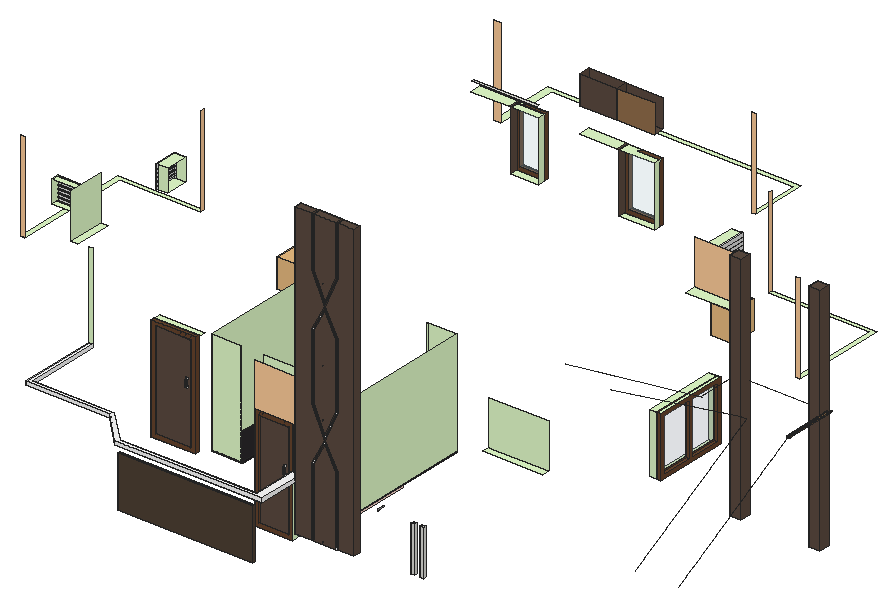
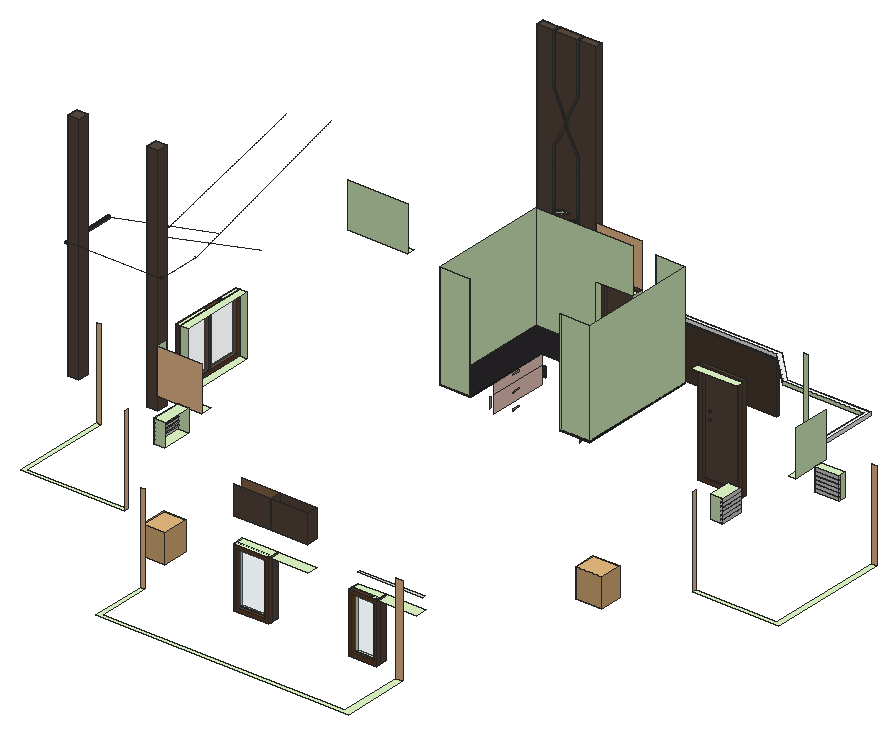
# SketchUp Ruby script. Lengths in inches.
U = 1.inch
M = Sketchup.active_model
def pt(a) = Geom::Point3d.new(a.map { |v| v * U })
def face(e, loops, mat)
  f = e.add_face(loops[0].map { |a| pt(a) })
  loops[1..].each { |l| e.add_face(l.map { |a| pt(a) }).erase! }
  f.material = f.back_material = mat if mat
  f
end
# faces: each face lists its corners as indices into pts; further lists are holes
def faces(e, pts, list, mat = nil) = list.each { |f| face(e, (f[0].is_a?(Array) ? f : [f]).map { |l| l.map { |i| pts[i] } }, mat) }
# xy, xz, yz: faces in a plane at the given z, y or x. An outline is a flat list of corners, or four numbers for a rectangle; further outlines are holes
def ring(l) = l.size == 4 ? [[l[0], l[1]], [l[2], l[1]], [l[2], l[3]], [l[0], l[3]]] : l.each_slice(2).to_a
def flat(e, list, mat, &to3) = list.each { |f| face(e, (f[0].is_a?(Array) ? f : [f]).map { |l| ring(l).map { |u, v| to3.(u, v) } }, mat) }
def xy(e, z, list, mat = nil) = flat(e, list, mat) { |x, y| [x, y, z] }
def xz(e, y, list, mat = nil) = flat(e, list, mat) { |x, z| [x, y, z] }
def yz(e, x, list, mat = nil) = flat(e, list, mat) { |y, z| [x, y, z] }
def lines(e, pts, list) = list.each { |a, b| e.add_line(pt(pts[a]), pt(pts[b])) }
# prism: a flat outline (further loops are holes) pulled along v
def prism(e, loops, v, mat = nil)
  f = face(e, loops, mat); d = Geom::Vector3d.new(v.map { |x| x * U })
  f.pushpull(f.normal.samedirection?(d) ? d.length : -d.length)
end
def box(e, o, s, mat = nil) = prism(e, [[o, [o[0] + s[0], o[1], o[2]], [o[0] + s[0], o[1] + s[1], o[2]], [o[0], o[1] + s[1], o[2]]]], [0, 0, s[2]], mat)
def at(x, y, z, deg = 0) = Geom::Transformation.translation(pt([x, y, z])) * Geom::Transformation.rotation(ORIGIN, Z_AXIS, deg.degrees)
def axes(o, x, y, z) = Geom::Transformation.new([*x, 0, *y, 0, *z, 0, *pt(o).to_a, 1])
def part(name) = M.definitions.add(name)
# library, detail: a bought-in or finely detailed component or shape, given as its bounding box
def library(name, o, s) = part(name).tap { |d| box(d.entities, o, s) }
def detail(e, o, s) = box(e.add_group.entities, o, s)
def put(e, d, t, mat = nil) = e.add_instance(d, t).tap { |i| i.material = mat if mat }
def group(e, t, mat = nil) = e.add_group.tap { |g| g.transformation = t; g.material = mat if mat }.entities
root = M.entities
M.materials.add("Asphalt_01_1K").color = [79, 65, 53]
M.materials.add("B01_Ivory_Dust").color = [255, 217, 206]
M.materials.add("C02_Golden_Beige").color = [255, 205, 155]
M.materials.add("F01_Seafoam_Drift").color = [229, 255, 204]
M.materials.add("Glass_Basic_01").color = [161, 173, 186]
M.materials["Glass_Basic_01"].alpha = 0.25
M.materials.add("Glass_Safety_01").color = [204, 235, 244]
M.materials["Glass_Safety_01"].alpha = 0.25
M.materials.add("M00_Soft_Cloud").color = [255, 255, 255]
M.materials.add("M01_Silver_Fog").color = [224, 224, 224]
M.materials.add("M03_Pewter_Shine").color = [168, 168, 168]
M.materials.add("M06_Steel_Smoke").color = [86, 86, 86]
M.materials.add("M08_Obsidian_Black").color = [30, 30, 30]
M.materials.add("M09_Shadow_Night").color = [0, 0, 0]
M.materials.add("Marble_07_1K").color = [36, 34, 36]
M.materials.add("Metal_06_1K").color = [238, 236, 231]
M.materials.add("Plywood_01_1K").color = [125, 96, 64]
M.materials.add("Wood_Floor_01_1K").color = [146, 111, 76]
M.materials.add("Wood_Floor_12_1K").color = [92, 75, 65]
M.materials.add("Wood_Veneer_15_1K").color = [103, 69, 45]
c1 = part("Group\#25")
xy(c1.entities,0,[[0,-3,30,0]],"Wood_Veneer_15_1K")
xy(c1.entities,3,[[3,-2.25,27,0]],"Wood_Floor_12_1K")
xy(c1.entities,3,[[3,-3,27,-2.25]],"Wood_Veneer_15_1K")
xy(c1.entities,81,[[3,-2.25,27,0]],"Wood_Floor_12_1K")
xy(c1.entities,81,[[3,-3,27,-2.25]],"Wood_Veneer_15_1K")
xy(c1.entities,84,[[0,-3,30,0]],"Wood_Veneer_15_1K")
xz(c1.entities,-3,[[[0,0,30,84],[3,3,27,81]]],"Wood_Veneer_15_1K")
xz(c1.entities,-2.25,[[3,3,27,81]],"Wood_Floor_12_1K")
xz(c1.entities,0,[[[0,0,30,84],[3,3,27,81]]],"Wood_Veneer_15_1K")
yz(c1.entities,0,[[-3,0,0,84]],"Wood_Veneer_15_1K")
yz(c1.entities,3,[[-2.25,3,0,81]],"Wood_Floor_12_1K")
yz(c1.entities,3,[[-3,3,-2.25,81]],"Wood_Veneer_15_1K")
yz(c1.entities,27,[[-2.25,3,0,81]],"Wood_Floor_12_1K")
yz(c1.entities,27,[[-3,3,-2.25,81]],"Wood_Veneer_15_1K")
yz(c1.entities,30,[[-3,0,0,84]],"Wood_Veneer_15_1K")
g1 = group(c1.entities,at(22.875,-2.25,50.47),"Metal_06_1K")
xy(g1,-5.5625,[[0,-0.48,1.25,0]],"Metal_06_1K")
xy(g1,-4.9375,[[0,-1.375,1.25,-0.48]],"Metal_06_1K")
xy(g1,-4.6875,[[0,-1.125,1.25,0]],"Metal_06_1K")
xy(g1,-4.6875,[[0,-1.375,1.25,-1.125]],"Wood_Veneer_15_1K")
xy(g1,0,[[0,-1.125,1.25,-0.5],[0,-0.5,1.25,0]],"Metal_06_1K")
xy(g1,0.25,[[0,-1.375,1.25,-1.125],[0,-1.125,1.25,-0.5]],"Metal_06_1K")
xy(g1,0.25,[[0,-0.5,1.25,0]],"Wood_Veneer_15_1K")
xy(g1,1.25,[[0,-0.5,1.25,0]],"Metal_06_1K")
xz(g1,-1.375,[[0,-4.9375,1.25,-4.6875],[0,-4.6875,1.25,0.25]],"Metal_06_1K")
xz(g1,-1.125,[[0,-4.6875,1.25,0],[0,0,1.25,0.25]],"Metal_06_1K")
xz(g1,-0.5,[[0,0.25,1.25,1.25]],"Metal_06_1K")
xz(g1,-0.5,[[0,0,1.25,0.25]],"Wood_Veneer_15_1K")
xz(g1,-0.48,[[0,-5.5625,1.25,-4.9375]],"Metal_06_1K")
xz(g1,0,[[0,0.25,1.25,1.25]],"Metal_06_1K")
xz(g1,0,[[0,-5.5625,1.25,-4.6875],[0,0,1.25,0.25]],"Wood_Veneer_15_1K")
yz(g1,0,[[-0.48,-5.5625,-0.48,-4.9375,-1.375,-4.9375,-1.375,-4.6875,0,-4.6875,0,-5.5625],[-1.375,-4.6875,-1.125,0.25],[-1.125,0,-0.5,0.25],[-0.5,0,0,0.25],[-0.5,0.25,0,1.25]],"Metal_06_1K")
yz(g1,1.25,[[-0.48,-5.5625,0,-5.5625,0,-4.6875,-1.375,-4.6875,-1.375,-4.9375,-0.48,-4.9375],[-1.375,-4.6875,-1.125,0.25],[-1.125,0,-0.5,0.25],[-0.5,0,0,0.25],[-0.5,0.25,0,1.25]],"Metal_06_1K")
c2 = part("Group\#51")
box(c2.entities,[0,0,-60],[9,9,187])
c3 = part("Group\#15")
box(c3.entities,[0,0,0],[5.9375,1,0.1875],"M03_Pewter_Shine")
c4 = part("Group\#49")
box(c4.entities,[2.9375,2.5,0],[1.8125,1.9375,1.6875],"M09_Shadow_Night")
c5 = part("Group\#58")
xy(c5.entities,0,[[-0.5,0,1.125,43.8125]],"M00_Soft_Cloud")
c6 = part("Group\#67")
box(c6.entities,[0,-2.3125,0],[2.875,2.3125,36.5625])
c7 = library("Hospital Sink 001",[-10.61,-17.4375,27.15],[21.22,17.43,22.96])
c8 = part("Group\#13")
box(c8.entities,[0,0,0],[1.125,8.25,0.1875],"M03_Pewter_Shine")
c9 = part("Group\#17")
xy(c9.entities,0,[[0,0,1.3125,6.9375]],"M06_Steel_Smoke")
c10 = part("Group\#16")
box(c10.entities,[0,0,0],[1.1875,8,0.25],"M03_Pewter_Shine")
c11 = part("Group\#14")
box(c11.entities,[0,0,0],[5.9375,1,0.1875],"M03_Pewter_Shine")
c12 = part("Group\#12")
box(c12.entities,[0,0,0],[5.9375,1,0.1875],"M03_Pewter_Shine")
c13 = part("Group\#28")
xy(c13.entities,0,[[0,0,28.0625,3]],"Wood_Veneer_15_1K")
xy(c13.entities,3,[[3,0,25.0625,3]],"Wood_Veneer_15_1K")
xy(c13.entities,45,[[3,0,25.0625,3]],"Wood_Veneer_15_1K")
xy(c13.entities,48,[[0,0,28.0625,3]],"Wood_Veneer_15_1K")
xz(c13.entities,0,[[3,3,25.0625,45]],"Glass_Safety_01")
xz(c13.entities,0,[[[0,0,28.0625,48],[3,3,25.0625,45]]],"Wood_Veneer_15_1K")
xz(c13.entities,3,[[[0,0,28.0625,48],[3,3,25.0625,45]]],"Wood_Veneer_15_1K")
yz(c13.entities,0,[[0,0,3,48]],"Wood_Veneer_15_1K")
yz(c13.entities,3,[[0,3,3,45]],"Wood_Veneer_15_1K")
yz(c13.entities,25.0625,[[0,3,3,45]],"Wood_Veneer_15_1K")
yz(c13.entities,28.0625,[[0,0,3,48]],"Wood_Veneer_15_1K")
c14 = part("Group\#27")
xy(c14.entities,0,[[0,0,3,60]],"Wood_Veneer_15_1K")
xy(c14.entities,3,[[0,3,3,29],[0,29,3,31],[0,31,3,57]],"Wood_Veneer_15_1K")
xy(c14.entities,45,[[0,3,3,29],[0,31,3,57]],"Wood_Veneer_15_1K")
xy(c14.entities,48,[[0,0,3,60]],"Wood_Veneer_15_1K")
xz(c14.entities,0,[[0,0,3,48]],"Wood_Veneer_15_1K")
xz(c14.entities,3,[[0,3,3,45]],"Wood_Veneer_15_1K")
xz(c14.entities,29,[[0,3,3,45]],"Wood_Veneer_15_1K")
xz(c14.entities,31,[[0,3,3,45]],"Wood_Veneer_15_1K")
xz(c14.entities,57,[[0,3,3,45]],"Wood_Veneer_15_1K")
xz(c14.entities,60,[[0,0,3,48]],"Wood_Veneer_15_1K")
yz(c14.entities,0,[[3,3,29,45],[31,3,57,45]],"Glass_Basic_01")
yz(c14.entities,0,[[[0,0,60,48],[3,3,57,3,57,45,31,45,31,3,29,3,29,45,3,45]]],"Wood_Veneer_15_1K")
yz(c14.entities,3,[[[0,0,60,48],[3,3,3,45,29,45,29,3,31,3,31,45,57,45,57,3]]],"Wood_Veneer_15_1K")
c15 = part("Group\#29")
xy(c15.entities,0,[[0,0,1,24]])
xy(c15.entities,2.6,[[0,0,1,24]])
xy(c15.entities,3,[[0,0,1,24]])
xy(c15.entities,5.6,[[0,0,1,24]])
xy(c15.entities,6,[[0,0,1,24]])
xy(c15.entities,8.6,[[0,0,1,24]])
xy(c15.entities,9,[[0,0,1,24]])
xy(c15.entities,11.6,[[0,0,1,24]])
xy(c15.entities,12,[[0,0,1,24]])
xy(c15.entities,14.6,[[0,0,1,24]])
xy(c15.entities,15,[[0,0,1,24]])
xy(c15.entities,18,[[0,0,1,24]])
xz(c15.entities,0,[[0,0,1,2.6],[0,3,1,5.6],[0,6,1,8.6],[0,9,1,11.6],[0,12,1,14.6],
  [0,15,1,18]])
xz(c15.entities,24,[[0,0,1,2.6],[0,3,1,5.6],[0,6,1,8.6],[0,9,1,11.6],[0,12,1,14.6],
  [0,15,1,18]])
yz(c15.entities,0,[[0,2.6,24,3],[0,5.6,24,6],[0,8.6,24,9],[0,11.6,24,12],[0,14.6,24,15]])
yz(c15.entities,1,[[0,0,24,2.6],[0,3,24,5.6],[0,6,24,8.6],[0,9,24,11.6],[0,12,24,14.6],
  [0,15,24,18]])
xy(root,23,[[1767.92,714.6875,1797.92,723.6875]],"Wood_Floor_12_1K")
xy(root,33.35,[[1804.92,714.6875,1851.8125,715.3125]],"F01_Seafoam_Drift")
xy(root,57,[[1797.92,723.6875,1797.92,747.03,1797.9375,747.22,1797.97,747.41,1798.04,747.59,1798.08,747.6875,1821.8125,747.6875,1821.8125,819.65,1821.81,819.65,1821.96,819.68,1822.1,819.6875,1845.8125,819.6875,1845.8125,723.6875],[1797.92,747.03,1797.9375,747.22,1797.97,747.41,1798.04,747.59,1798.08,747.6875,1797.92,747.6875]],"B01_Ivory_Dust")
xy(root,57,[[1798.08,747.6875,1798.12,747.76,1798.23,747.92,1798.36,748.07,1798.5,748.2,1798.66,748.3,1798.83,748.39,1799.02,748.45,1799.2,748.49,1799.4,748.5,1821,748.5,1821,747.6875],[1821,747.6875,1821.8125,795.6875],[1821,795.6875,1821,818.59,1821.01,818.73,1821.04,818.87,1821.08,819.01,1821.15,819.14,1821.23,819.26,1821.32,819.37,1821.43,819.46,1821.55,819.54,1821.68,819.6,1821.8125,819.65,1821.8125,795.6875],[1821.81,819.65,1821.96,819.68,1822.1,819.6875,1821.8125,819.6875,1821.8125,819.65]],"Marble_07_1K")
xy(root,58,[[1725.8125,723.6875,1725.8125,819.6875,1748.87,819.6875,1749.1,819.67,1749.32,819.63,1749.54,819.55,1749.75,819.45,1749.8125,819.41,1749.8125,723.73,1749.79,723.73,1749.64,723.7,1749.5,723.6875],[1749.5,723.6875,1749.8125,723.6875,1749.8125,723.73,1749.79,723.73,1749.64,723.7]],"B01_Ivory_Dust")
xy(root,58,[[1959.8125,869.89,1968.8125,929.89],[1651.0625,1117.375,1673.1875,1126.375],[1737.77,1117.375,1765.83,1126.375]],"F01_Seafoam_Drift")
xy(root,58,[[1797.92,723.6875,1845.8125,723.6875,1845.8125,819.6875,1822.1,819.6875,1821.96,819.68,1821.81,819.65,1821.68,819.6,1821.55,819.54,1821.43,819.46,1821.32,819.37,1821.23,819.26,1821.15,819.14,1821.08,819.01,1821.04,818.87,1821.01,818.73,1821,818.59,1821,748.5,1799.4,748.5,1799.2,748.49,1799.02,748.45,1798.83,748.39,1798.66,748.3,1798.5,748.2,1798.36,748.07,1798.23,747.92,1798.12,747.76,1798.04,747.59,1797.97,747.41,1797.9375,747.22,1797.92,747.03],[1749.8125,723.73,1749.8125,747.6875,1750.625,747.6875,1750.625,724.82,1750.62,724.67,1750.59,724.52,1750.54,724.38,1750.47,724.25,1750.39,724.13,1750.29,724.02,1750.18,723.92,1750.06,723.84,1749.93,723.77],[1749.8125,747.6875,1750.625,771.6875],[1749.8125,771.6875,1750.625,795.6875],[1749.8125,795.6875,1749.8125,819.41,1749.9375,819.32,1750.11,819.17,1750.26,819,1750.39,818.81,1750.49,818.6,1750.57,818.38,1750.61,818.16,1750.625,817.93,1750.625,795.6875],
  [1749.8125,819.41,1749.8125,819.6875,1748.87,819.6875,1749.1,819.67,1749.32,819.63,1749.54,819.55,1749.75,819.45]],"Marble_07_1K")
xy(root,59,[[1725.8125,723.6875,1749.5,723.6875,1749.64,723.7,1749.79,723.73,1749.93,723.77,1750.06,723.84,1750.18,723.92,1750.29,724.02,1750.39,724.13,1750.47,724.25,1750.54,724.38,1750.59,724.52,1750.62,724.67,1750.625,724.82,1750.625,817.93,1750.61,818.16,1750.57,818.38,1750.49,818.6,1750.39,818.81,1750.26,819,1750.11,819.17,1749.9375,819.32,1749.75,819.45,1749.54,819.55,1749.32,819.63,1749.1,819.67,1748.87,819.6875,1725.8125,819.6875]],"Marble_07_1K")
xy(root,70,[[1687.27,675.6875,1662.78,700.375,1596.1,700.375,1596.1,763.375,1599.1,763.375,1599.1,703.375,1664.03,703.375,1688.52,678.6875,1797.92,678.6875,1797.92,714.6875,1804.92,714.6875,1804.92,675.6875],[1473.8125,847.375,1477.8125,847.375,1477.8125,941.875,1542.8125,941.875,1542.8125,944.875,1473.8125,944.875],[1965.8125,1009.375,1968.8125,1009.375,1968.8125,1086,1884.8125,1086,1884.8125,1083,1965.8125,1083],[1613.1875,1147.375,1619.1875,1147.375,1619.1875,1198.375,1812.8125,1198.375,1812.8125,1156.375,1815.8125,1156.375,1815.8125,1201.375,1613.1875,1201.375]],"F01_Seafoam_Drift")
xy(root,73,[[1687.27,675.6875,1804.92,675.6875,1804.92,714.6875,1797.92,714.6875,1797.92,678.6875,1688.52,678.6875,1664.03,703.375,1599.1,703.375,1599.1,763.375,1596.1,763.375,1596.1,700.375,1662.78,700.375]],"M00_Soft_Cloud")
xy(root,106,[[1767.92,714.6875,1797.92,723.6875],[1911.8125,763,1959.8125,769],[1645.59,763.375,1681.59,772.375],[1542.8125,811.375,1548.8125,841.375],[1504.12,841.375,1523.47,847.375],
  [1959.8125,869.89,1968.8125,929.89],[1542.8125,897.17,1551.8125,915.375],[1875.8125,1033.59,1884.8125,1057.59],[1619.1875,1117.375,1649.1875,1126.375],[1651.0625,1117.375,1673.1875,1126.375],
  [1705.83,1117.375,1735.83,1126.375],[1737.77,1117.375,1765.83,1126.375]],"F01_Seafoam_Drift")
xy(root,106,[[1649.1875,1117.375,1651.0625,1126.375],[1735.83,1117.375,1737.77,1126.375]],"Wood_Floor_12_1K")
xy(root,106.25,[[1884.8125,1000.375,1920.8125,1009.375]],"F01_Seafoam_Drift")
xy(root,123,[[1993.5,912.38,1994.68,912.38,1994.68,912.82,1994.875,912.82,1994.875,914,1993.5,914],[1994.68,912.38,1994.875,912.82],[2066.875,912.38,2067.19,912.82],[2067.19,912.38,2068.375,912.38,2068.375,914,2066.875,914,2066.875,912.82,2067.19,912.82]])
xy(root,124,[[1504.12,841.375,1523.47,847.375],[1542.8125,897.17,1551.8125,915.375],[1875.8125,1033.59,1884.8125,1057.59]],"F01_Seafoam_Drift")
xy(root,126.3125,[[1705.83,1117.375,1735.83,1126.375],[1735.83,1117.375,1765.83,1126.375]],"Wood_Floor_12_1K")
xz(root,675.6875,[[1687.27,70,1804.92,73]],"M00_Soft_Cloud")
xz(root,678.6875,[[1688.52,70,1797.92,73]],"M00_Soft_Cloud")
xz(root,700.375,[[1596.1,70,1662.78,73]],"M00_Soft_Cloud")
xz(root,703.375,[[1599.1,70,1664.03,73]],"F01_Seafoam_Drift")
xz(root,714.6875,[[1797.92,73,1804.92,73,1804.92,142,1767.92,142,1767.92,106,1797.92,106]],"C02_Golden_Beige")
xz(root,714.6875,[[1804.92,33.35,1851.8125,142],[1797.92,70,1804.92,73]],"F01_Seafoam_Drift")
xz(root,723.6875,[[1749.5,58,1749.8125,142],[1797.92,58,1797.92,106,1767.92,106,1767.92,142,1845.8125,142,1845.8125,58],[1725.8125,59,1749.5,142]],"F01_Seafoam_Drift")
xz(root,723.6875,[[1797.92,57,1845.8125,58],[1725.8125,58,1749.5,59]],"Marble_07_1K")
xz(root,748.5,[[1799.4,57,1821,58]],"Marble_07_1K")
xz(root,763.375,[[1596.1,70,1599.1,73],[1596.1,73,1599.1,142]],"F01_Seafoam_Drift")
xz(root,769,[[1911.8125,106,1959.8125,142]],"F01_Seafoam_Drift")
xz(root,819.6875,[[1821.8125,57,1822.1,142],[1748.87,58,1749.8125,142],[1822.1,58,1845.8125,142],[1725.8125,59,1748.87,142]],"F01_Seafoam_Drift")
xz(root,819.6875,[[1822.1,57,1845.8125,58],[1725.8125,58,1748.87,59]],"Marble_07_1K")
xz(root,847.375,[[1473.8125,70,1477.8125,142]],"C02_Golden_Beige")
xz(root,869.89,[[1959.8125,58,1968.8125,106]],"F01_Seafoam_Drift")
xz(root,897.17,[[1542.8125,106,1551.8125,124]],"F01_Seafoam_Drift")
xz(root,915.375,[[1542.8125,106,1551.8125,124]],"F01_Seafoam_Drift")
xz(root,929.89,[[1959.8125,58,1968.8125,106]],"F01_Seafoam_Drift")
xz(root,1009.375,[[1965.8125,70,1968.8125,142],[1884.8125,106.25,1920.8125,142]],"C02_Golden_Beige")
xz(root,1033.59,[[1875.8125,106,1884.8125,124]],"F01_Seafoam_Drift")
xz(root,1057.59,[[1875.8125,106,1884.8125,124]],"F01_Seafoam_Drift")
xz(root,1117.375,[[1735.83,126.3125,1765.83,149]],"Wood_Floor_01_1K")
xz(root,1117.375,[[1705.83,126.3125,1735.83,149]],"Wood_Floor_12_1K")
xz(root,1126.375,[[1705.83,126.3125,1735.83,149],[1735.83,126.3125,1765.83,149]],"Wood_Floor_12_1K")
xz(root,1147.375,[[1613.1875,70,1619.1875,142]],"C02_Golden_Beige")
xz(root,1156.375,[[1812.8125,70,1815.8125,142]],"C02_Golden_Beige")
yz(root,1504.12,[[841.375,106,847.375,124]],"F01_Seafoam_Drift")
yz(root,1523.47,[[841.375,106,847.375,124]],"F01_Seafoam_Drift")
yz(root,1542.8125,[[941.875,70,944.875,142]],"C02_Golden_Beige")
yz(root,1542.8125,[[811.375,106,841.375,142]],"F01_Seafoam_Drift")
yz(root,1596.1,[[700.375,70,763.375,73]],"M00_Soft_Cloud")
yz(root,1599.1,[[703.375,70,763.375,73]],"M00_Soft_Cloud")
yz(root,1651.0625,[[1117.375,58,1126.375,106]],"Wood_Floor_12_1K")
yz(root,1673.1875,[[1117.375,58,1126.375,106]],"F01_Seafoam_Drift")
yz(root,1705.83,[[1117.375,126.3125,1126.375,149]],"Wood_Floor_12_1K")
yz(root,1725.8125,[[723.6875,59,819.6875,142]],"F01_Seafoam_Drift")
yz(root,1725.8125,[[723.6875,58,819.6875,59]],"Marble_07_1K")
yz(root,1735.83,[[1117.375,126.3125,1126.375,149]],"Wood_Floor_12_1K")
yz(root,1737.77,[[1117.375,58,1126.375,106]],"Wood_Floor_12_1K")
yz(root,1750.625,[[724.82,58,817.93,59]],"Marble_07_1K")
yz(root,1765.83,[[1117.375,58,1126.375,106]],"F01_Seafoam_Drift")
yz(root,1767.92,[[714.6875,23,723.6875,106]],"F01_Seafoam_Drift")
yz(root,1797.92,[[714.6875,23,723.6875,106]],"F01_Seafoam_Drift")
yz(root,1797.92,[[678.6875,70,714.6875,73]],"M00_Soft_Cloud")
yz(root,1797.92,[[723.6875,57,747.03,58]],"Marble_07_1K")
yz(root,1804.92,[[675.6875,70,714.6875,73]],"M00_Soft_Cloud")
yz(root,1821,[[748.5,57,818.59,58]],"Marble_07_1K")
yz(root,1821.8125,[[747.6875,34,795.6875,47.875],[747.6875,47.875,795.6875,57]],"B01_Ivory_Dust")
yz(root,1845.8125,[[723.6875,58,819.6875,142]],"F01_Seafoam_Drift")
yz(root,1845.8125,[[723.6875,57,819.6875,58]],"Marble_07_1K")
yz(root,1884.8125,[[1083,70,1086,142]],"C02_Golden_Beige")
yz(root,1920.8125,[[1000.375,106.25,1009.375,142]],"F01_Seafoam_Drift")
p = [[1797.92,747.03,58],[1797.9375,747.22,58],[1797.9375,747.22,57],[1797.92,747.03,57],[1797.97,747.41,58],[1797.97,747.41,57],
  [1798.04,747.59,58],[1798.04,747.59,57],[1798.12,747.76,58],[1798.12,747.76,57],[1798.08,747.6875,57],[1798.23,747.92,58],
  [1798.23,747.92,57],[1798.36,748.07,58],[1798.36,748.07,57],[1798.5,748.2,58],[1798.5,748.2,57],[1798.66,748.3,58],
  [1798.66,748.3,57],[1798.83,748.39,58],[1798.83,748.39,57],[1799.02,748.45,58],[1799.02,748.45,57],[1799.2,748.49,58],
  [1799.2,748.49,57],[1799.4,748.5,58],[1799.4,748.5,57],[1821,818.59,58],[1821.01,818.73,58],[1821.01,818.73,57],
  [1821,818.59,57],[1821.04,818.87,58],[1821.04,818.87,57],[1821.08,819.01,58],[1821.08,819.01,57],[1821.15,819.14,58],
  [1821.15,819.14,57],[1821.23,819.26,58],[1821.23,819.26,57],[1821.32,819.37,58],[1821.32,819.37,57],[1821.43,819.46,58],
  [1821.43,819.46,57],[1821.55,819.54,58],[1821.55,819.54,57],[1821.68,819.6,58],[1821.68,819.6,57],[1821.81,819.65,58],
  [1821.81,819.65,57],[1821.8125,819.65,57],[1821.96,819.68,58],[1821.96,819.68,57],[1822.1,819.6875,58],[1822.1,819.6875,57],
  [1749.64,723.7,59],[1749.5,723.6875,59],[1749.5,723.6875,58],[1749.64,723.7,58],[1749.79,723.73,59],[1749.79,723.73,58],
  [1749.93,723.77,59],[1749.8125,723.73,58],[1749.93,723.77,58],[1750.06,723.84,59],[1750.06,723.84,58],[1750.18,723.92,59],
  [1750.18,723.92,58],[1750.29,724.02,59],[1750.29,724.02,58],[1750.39,724.13,59],[1750.39,724.13,58],[1750.47,724.25,59],
  [1750.47,724.25,58],[1750.54,724.38,59],[1750.54,724.38,58],[1750.59,724.52,59],[1750.59,724.52,58],[1750.62,724.67,59],
  [1750.62,724.67,58],[1750.625,724.82,59],[1750.625,724.82,58],[1750.61,818.16,59],[1750.625,817.93,59],[1750.625,817.93,58],
  [1750.61,818.16,58],[1750.57,818.38,59],[1750.57,818.38,58],[1750.49,818.6,59],[1750.49,818.6,58],[1750.39,818.81,59],
  [1750.39,818.81,58],[1750.26,819,59],[1750.26,819,58],[1750.11,819.17,59],[1750.11,819.17,58],[1749.9375,819.32,59],
  [1749.9375,819.32,58],[1749.75,819.45,59],[1749.8125,819.41,58],[1749.75,819.45,58],[1749.54,819.55,59],[1749.54,819.55,58],
  [1749.1,819.67,59],[1749.32,819.63,59],[1749.32,819.63,58],[1749.1,819.67,58],[1748.87,819.6875,59],[1748.87,819.6875,58],
  [1662.78,700.375,70],[1687.27,675.6875,70],[1687.27,675.6875,73],[1662.78,700.375,73],[1688.52,678.6875,70],[1664.03,703.375,70],
  [1664.03,703.375,73],[1688.52,678.6875,73],[2067.78,912.38,122.1],[2067.78,913.41,122.1],[2068.07,913.7,122],[2068.07,912.38,122],
  [2068.07,873.26,122],[2067.78,873.23,122.1],[2068.97,873.23,122.1],[2068.68,873.26,122],[2068.68,912.38,122],[2068.68,914.31,122],
  [2068.97,914.6,122.1],[2068.97,912.38,122.1],[2068.375,914,121.96],[2068.375,912.38,121.96],[2068.375,873.27,121.96],[2067.54,912.38,122.27],
  [2067.54,913.17,122.27],[2067.54,873.19,122.27],[2069.21,873.19,122.27],[2069.21,914.84,122.27],[2069.21,912.38,122.27],[2067.35,873.14,122.48],
  [2067.35,912.38,122.48],[2067.35,912.98,122.48],[2069.4,873.14,122.48],[2069.4,915.03,122.48],[2069.4,912.38,122.48],[2067.23,912.38,122.73],
  [2067.23,912.86,122.73],[2067.23,873.07,122.73],[2069.52,873.07,122.73],[2069.52,915.15,122.73],[2069.52,912.38,122.73],[2067.19,873,123],
  [2067.19,912.38,123],[2067.19,912.82,123],[2069.56,915.1875,123],[2069.56,912.38,123],[2069.56,873,123],[2067.23,912.38,123.27],
  [2067.23,912.86,123.27],[2067.23,872.9375,123.27],[2069.52,915.15,123.27],[2069.52,912.38,123.27],[2069.52,872.9375,123.27],[2067.35,872.87,123.52],
  [2067.35,912.38,123.52],[2067.35,912.98,123.52],[2069.4,915.03,123.52],[2069.4,912.38,123.52],[2069.4,872.87,123.52],[2067.54,872.82,123.73],
  [2067.54,912.38,123.73],[2067.54,913.17,123.73],[2069.21,872.82,123.73],[2069.21,914.84,123.73],[2069.21,912.38,123.73],[2067.78,872.78,123.9],
  [2067.78,912.38,123.9],[2067.78,913.41,123.9],[2068.97,872.78,123.9],[2068.97,914.6,123.9],[2068.97,912.38,123.9],[2068.07,872.75,124],
  [2068.07,912.38,124],[2068.07,913.7,124],[2068.68,872.75,124],[2068.68,914.31,124],[2068.68,912.38,124],[2068.375,872.74,124.04],
  [2068.375,912.38,124.04],[2068.375,914,124.04],[2068.375,873,123],[1994.875,878.88,123],[1994.68,878.88,123],[2033.875,763,63],
  [2033.875,874.63,123],[2027.875,874.63,123],[2003.875,775.63,177],[2068.375,763,63],[2068.375,912.38,123],[2066.875,914,123],
  [1994.875,914,123],[1993.5,912.38,123],[1993.5,878.88,123],[1968.8125,774,184],[2066.875,873,123],[1765.83,1117.375,106],
  [1765.83,1117.09,106]]
faces(root,p,[[0,1,2,3],[1,4,5,2],[4,6,7,5],[6,8,9,10,7],[8,11,12,9],[11,13,14,12],[13,15,16,14],[15,17,18,16],
  [17,19,20,18],[19,21,22,20],[21,23,24,22],[23,25,26,24],[27,28,29,30],[28,31,32,29],[31,33,34,32],[33,35,36,34],
  [35,37,38,36],[37,39,40,38],[39,41,42,40],[41,43,44,42],[43,45,46,44],[45,47,48,49,46],[47,50,51,48],[50,52,53,51],
  [54,55,56,57],[58,54,57,59],[60,58,59,61,62],[63,60,62,64],[65,63,64,66],[67,65,66,68],[69,67,68,70],[71,69,70,72],
  [73,71,72,74],[75,73,74,76],[77,75,76,78],[79,77,78,80],[81,82,83,84],[85,81,84,86],[87,85,86,88],[89,87,88,90],
  [91,89,90,92],[93,91,92,94],[95,93,94,96],[97,95,96,98,99],[100,97,99,101],[102,103,104,105],[103,100,101,104],[106,102,105,107]],"Marble_07_1K")
faces(root,p,[[108,109,110,111]],"F01_Seafoam_Drift")
faces(root,p,[[112,113,114,115]],"M00_Soft_Cloud")
faces(root,p,[[116,117,118,119,120,121],[122,123,124,125,126,127],[119,118,128,129,130,120],[129,128,125,124,123,130],[131,132,117,116,121,133],[134,122,127,126,135,136],[133,137,138,139,132,131],[140,134,136,135,141,142],
  [143,144,139,138,137,145],[146,140,142,141,147,148],[145,149,150,151,144,143],[148,147,152,153,154,146],[155,156,151,150,149,157],[153,152,158,159,160,154],[157,161,162,163,156,155],[159,158,164,165,166,160],
  [161,167,168,169,163,162],[170,166,165,164,171,172],[167,173,174,175,169,168],[176,170,172,171,177,178],[173,179,180,181,175,174],[182,176,178,177,183,184],[179,185,186,187,181,180],[185,182,184,183,187,186]],"Plywood_01_1K")
lines(root,p,[[188,149],[189,190],[191,192],[192,193],[193,194],[195,188],[188,196],[197,198],[199,200],[200,201],[149,202],[190,200],
  [203,204]])
put(root,c1,at(1767.92,717.6875,23),"M00_Soft_Cloud")
put(root,c1,axes([1645.59,766.375,23],[1.2,0,0],[0,1,0],[0,0,1]),"M00_Soft_Cloud")
g2 = group(root,at(1690.77,675.6875,25.67),"Asphalt_01_1K")
box(g2,[0,-2.0625,0],[108.3125,2.0625,40.5625])
put(root,c2,at(2059.375,905,87),"Wood_Floor_12_1K")
put(root,c2,at(1996.04,904.82,87),"Wood_Floor_12_1K")
put(root,c3,axes([1821.8125,776.71,28.33],[0,-1,0],[0,0,1],[-1,0,0]),"M03_Pewter_Shine")
g3 = group(root,at(1804.92,708.6875,33.35),"Wood_Veneer_15_1K")
xy(g3,0,[[0,0,13.58,6],[34.08,0,46.9,6]],"Wood_Floor_12_1K")
xy(g3,234.71,[[0,0,13.58,6],[14.88,0,32.78,6],[34.08,0,46.9,6]],"Wood_Floor_12_1K")
xz(g3,0,[[13.58,0,14.88,0,14.88,55.45,23.83,72.4,32.78,55.45,32.78,0,34.08,0,34.08,55.66,23.83,75.09,13.58,55.66],[[23.83,75.09,34.08,98.59,34.08,151.57,23.83,170.99,13.58,151.57,13.58,98.59],[23.83,78.25,14.88,98.77,14.88,151.35,23.83,168.31,32.78,151.35,32.78,98.77]],[23.83,170.99,34.08,194.5,34.08,234.71,32.78,234.71,32.78,194.68,23.83,174.16,14.88,194.68,14.88,234.71,13.58,234.71,13.58,194.5]],"M00_Soft_Cloud")
xz(g3,0,[[0,0,13.58,0,13.58,55.66,23.83,75.09,13.58,98.59,13.58,151.57,23.83,170.99,34.08,151.57,34.08,98.59,23.83,75.09,34.08,55.66,34.08,0,46.9,0,46.9,234.71,34.08,234.71,34.08,194.5,23.83,170.99,13.58,194.5,13.58,234.71,0,234.71],[14.88,0,32.78,0,32.78,55.45,23.83,72.4,14.88,55.45],[23.83,78.25,32.78,98.77,32.78,151.35,23.83,168.31,14.88,151.35,14.88,98.77],[23.83,174.16,32.78,194.68,32.78,234.71,14.88,234.71,14.88,194.68]],"Wood_Floor_12_1K")
xz(g3,6,[[0,0,0,234.71,13.58,234.71,13.58,194.5,23.83,170.99,34.08,194.5,34.08,234.71,46.9,234.71,46.9,0,34.08,0,34.08,55.66,23.83,75.09,34.08,98.59,34.08,151.57,23.83,170.99,13.58,151.57,13.58,98.59,23.83,75.09,13.58,55.66,13.58,0],[14.88,1.05,14.88,55.45,23.83,72.4,32.78,55.45,32.78,1.05],[23.83,78.25,14.88,98.77,14.88,151.35,23.83,168.31,32.78,151.35,32.78,98.77],[23.83,174.16,14.88,194.68,14.88,234.71,32.78,234.71,32.78,194.68]],"Wood_Floor_12_1K")
yz(g3,0,[[0,0,6,234.71]],"Wood_Floor_12_1K")
yz(g3,13.58,[[0,0,6,55.66],[0,98.59,6,138.8],[0,138.8,6,151.57],[0,194.5,6,234.71]],"Wood_Floor_12_1K")
yz(g3,14.88,[[0,1.05,6,55.45],[0,98.77,6,138.8],[0,138.8,6,151.35],[0,194.68,6,234.71]],"Wood_Floor_12_1K")
yz(g3,32.78,[[0,1.05,6,55.45],[0,98.77,6,138.8],[0,138.8,6,151.35],[0,194.68,6,234.71]],"Wood_Floor_12_1K")
yz(g3,34.08,[[0,0,6,55.66],[0,98.59,6,138.8],[0,138.8,6,151.57],[0,194.5,6,234.71]],"Wood_Floor_12_1K")
yz(g3,46.9,[[0,0,6,234.71]],"Wood_Floor_12_1K")
p = [[14.88,0,55.45],[23.83,0,72.4],[23.83,6,72.4],[14.88,6,55.45],[32.78,0,55.45],[32.78,6,55.45],
  [23.83,0,75.09],[13.58,0,55.66],[13.58,6,55.66],[23.83,6,75.09],[34.08,0,55.66],[34.08,6,55.66],
  [13.58,0,98.59],[13.58,6,98.59],[34.08,0,98.59],[34.08,6,98.59],[23.83,0,78.25],[14.88,0,98.77],
  [14.88,6,98.77],[23.83,6,78.25],[32.78,0,98.77],[32.78,6,98.77],[14.88,0,151.35],[23.83,0,168.31],
  [23.83,6,168.31],[14.88,6,151.35],[32.78,0,151.35],[32.78,6,151.35],[23.83,0,170.99],[13.58,0,151.57],
  [13.58,6,151.57],[23.83,6,170.99],[34.08,0,151.57],[34.08,6,151.57],[13.58,0,194.5],[13.58,6,194.5],
  [34.08,0,194.5],[34.08,6,194.5],[23.83,0,174.16],[14.88,0,194.68],[14.88,6,194.68],[23.83,6,174.16],
  [32.78,0,194.68],[32.78,6,194.68]]
faces(g3,p,[[0,1,2,3],[1,4,5,2],[6,7,8,9],[10,6,9,11],[12,6,9,13],[6,14,15,9],[16,17,18,19],[20,16,19,21],
  [22,23,24,25],[23,26,27,24],[28,29,30,31],[32,28,31,33],[34,28,31,35],[28,36,37,31],[38,39,40,41],[42,38,41,43]],"Wood_Floor_12_1K")
put(g3,c4,axes([19.68,6,167.45],[1,0,0],[0,0,0.80934],[0,-1,0]),"M08_Obsidian_Black")
put(g3,c4,axes([19.68,6,72.51],[1,0,0],[0,0,0.80934],[0,-1,0]),"M08_Obsidian_Black")
put(g3,c5,axes([23.04,0,1.23],[1,0,0],[0,0,0.80934],[0,-1,0]),"M00_Soft_Cloud")
put(g3,c5,axes([23.04,0,89.04],[1,0,0],[0,0,0.80934],[0,-1,0]),"M00_Soft_Cloud")
put(g3,c5,axes([23.04,0,127.85],[1,0,0],[0,0,0.80934],[0,-1,0]),"M00_Soft_Cloud")
put(g3,c5,axes([23.04,0,186.85],[1,0,0],[0,0,0.80934],[0,-1,0]),"M00_Soft_Cloud")
put(root,c6,at(1899.71,708.6875,38.72))
put(root,c6,at(1906.77,708.6875,38.72))
put(root,c7,at(1618.3,954.49,12.14))
put(root,c7,at(1874.09,1071.08,12.14,-90))
put(root,c8,axes([1821.8125,799.69,39.9],[0,-1,0],[0,0,1],[-1,0,0]),"F01_Seafoam_Drift")
put(root,c9,axes([1749.8125,743.625,40.35],[0,1,0],[0,0,1],[1,0,0]),"M06_Steel_Smoke")
put(root,c9,axes([1749.8125,749.3125,40.35],[0,1,0],[0,0,1],[1,0,0]),"M06_Steel_Smoke")
put(root,c9,axes([1749.8125,774.25,40.35],[0,1,0],[0,0,1],[1,0,0]),"M06_Steel_Smoke")
put(root,c9,axes([1749.8125,768.5625,40.35],[0,1,0],[0,0,1],[1,0,0]),"M06_Steel_Smoke")
put(root,c9,axes([1749.8125,792.5625,40.35],[0,1,0],[0,0,1],[1,0,0]),"M06_Steel_Smoke")
put(root,c9,axes([1749.8125,798.25,40.35],[0,1,0],[0,0,1],[1,0,0]),"M06_Steel_Smoke")
put(root,c10,axes([1819.5,747.6875,40.4],[-1,0,0],[0,0,1],[0,1,0]),"F01_Seafoam_Drift")
put(root,c11,axes([1821.8125,776.71,41.14],[0,-1,0],[0,0,1],[-1,0,0]),"M03_Pewter_Shine")
put(root,c12,axes([1821.8125,776.71,53.83],[0,-1,0],[0,0,1],[-1,0,0]),"M03_Pewter_Shine")
put(root,c13,at(1737.77,1123.375,58),"F01_Seafoam_Drift")
put(root,c14,at(1965.8125,869.89,58),"M00_Soft_Cloud")
put(root,c13,axes([1651.0625,1123.375,58],[0.78842,0,0],[0,1,0],[0,0,1]),"F01_Seafoam_Drift")
put(root,c15,axes([1523.45,846.375,106],[0,1,0],[-0.8056,0,0],[0,0,1]),"M01_Silver_Fog")
put(root,c15,at(1883.8125,1033.59,106),"M01_Silver_Fog")
put(root,c15,axes([1543.8125,915.37,106],[-1,0,0],[0,-0.76,0],[0,0,1]),"M01_Silver_Fog")
g4 = group(root,at(1620.58,1115.83,114.67))
xy(g4,0,[[0,0,52.32,2.32]])
